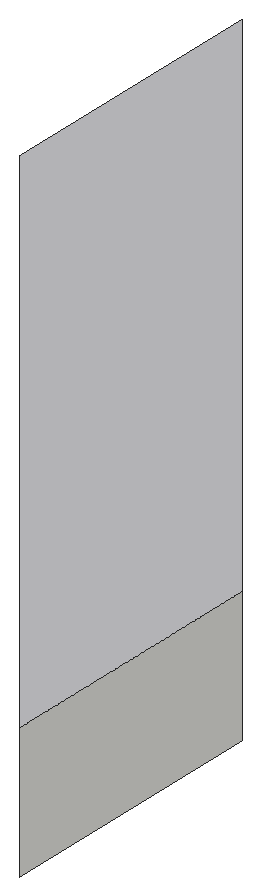
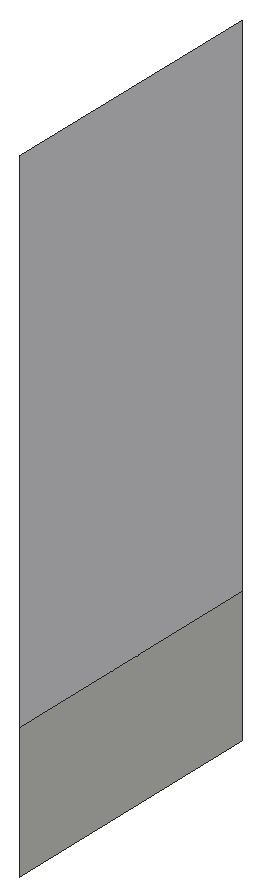
# SketchUp Ruby script. Lengths in inches.
U = 1.inch
M = Sketchup.active_model
def pt(a) = Geom::Point3d.new(a.map { |v| v * U })
def face(e, loops, mat)
  f = e.add_face(loops[0].map { |a| pt(a) })
  loops[1..].each { |l| e.add_face(l.map { |a| pt(a) }).erase! }
  f.material = f.back_material = mat if mat
  f
end
# faces: each face lists its corners as indices into pts; further lists are holes
def faces(e, pts, list, mat = nil) = list.each { |f| face(e, (f[0].is_a?(Array) ? f : [f]).map { |l| l.map { |i| pts[i] } }, mat) }
# xy, xz, yz: faces in a plane at the given z, y or x. An outline is a flat list of corners, or four numbers for a rectangle; further outlines are holes
def ring(l) = l.size == 4 ? [[l[0], l[1]], [l[2], l[1]], [l[2], l[3]], [l[0], l[3]]] : l.each_slice(2).to_a
def flat(e, list, mat, &to3) = list.each { |f| face(e, (f[0].is_a?(Array) ? f : [f]).map { |l| ring(l).map { |u, v| to3.(u, v) } }, mat) }
def xy(e, z, list, mat = nil) = flat(e, list, mat) { |x, y| [x, y, z] }
def xz(e, y, list, mat = nil) = flat(e, list, mat) { |x, z| [x, y, z] }
def yz(e, x, list, mat = nil) = flat(e, list, mat) { |y, z| [x, y, z] }
def lines(e, pts, list) = list.each { |a, b| e.add_line(pt(pts[a]), pt(pts[b])) }
# prism: a flat outline (further loops are holes) pulled along v
def prism(e, loops, v, mat = nil)
  f = face(e, loops, mat); d = Geom::Vector3d.new(v.map { |x| x * U })
  f.pushpull(f.normal.samedirection?(d) ? d.length : -d.length)
end
def box(e, o, s, mat = nil) = prism(e, [[o, [o[0] + s[0], o[1], o[2]], [o[0] + s[0], o[1] + s[1], o[2]], [o[0], o[1] + s[1], o[2]]]], [0, 0, s[2]], mat)
def at(x, y, z, deg = 0) = Geom::Transformation.translation(pt([x, y, z])) * Geom::Transformation.rotation(ORIGIN, Z_AXIS, deg.degrees)
def axes(o, x, y, z) = Geom::Transformation.new([*x, 0, *y, 0, *z, 0, *pt(o).to_a, 1])
def part(name) = M.definitions.add(name)
# library, detail: a bought-in or finely detailed component or shape, given as its bounding box
def library(name, o, s) = part(name).tap { |d| box(d.entities, o, s) }
def detail(e, o, s) = box(e.add_group.entities, o, s)
def put(e, d, t, mat = nil) = e.add_instance(d, t).tap { |i| i.material = mat if mat }
def group(e, t, mat = nil) = e.add_group.tap { |g| g.transformation = t; g.material = mat if mat }.entities
root = M.entities
M.materials.add("[Blinds Vertical Pattern]1").color = [239, 239, 242]
yz(root,315.3,[[96.24,0,111,7.1]])
yz(root,315.3,[[96.24,7.1,111,34.41]],"[Blinds Vertical Pattern]1")
